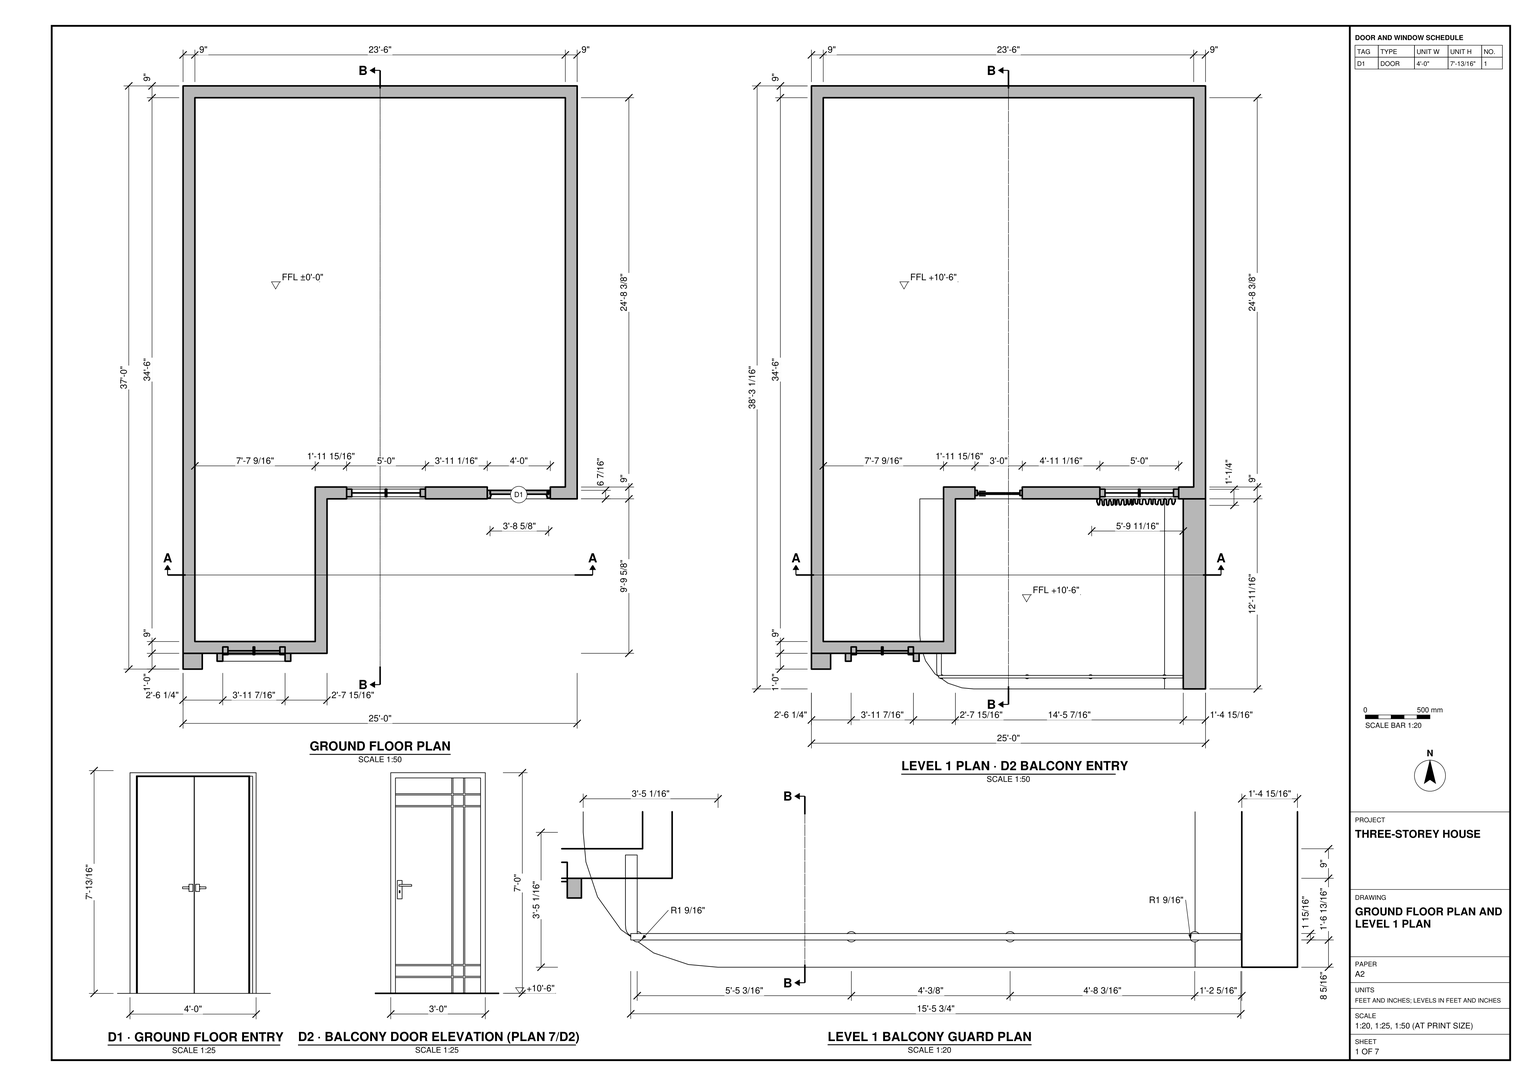
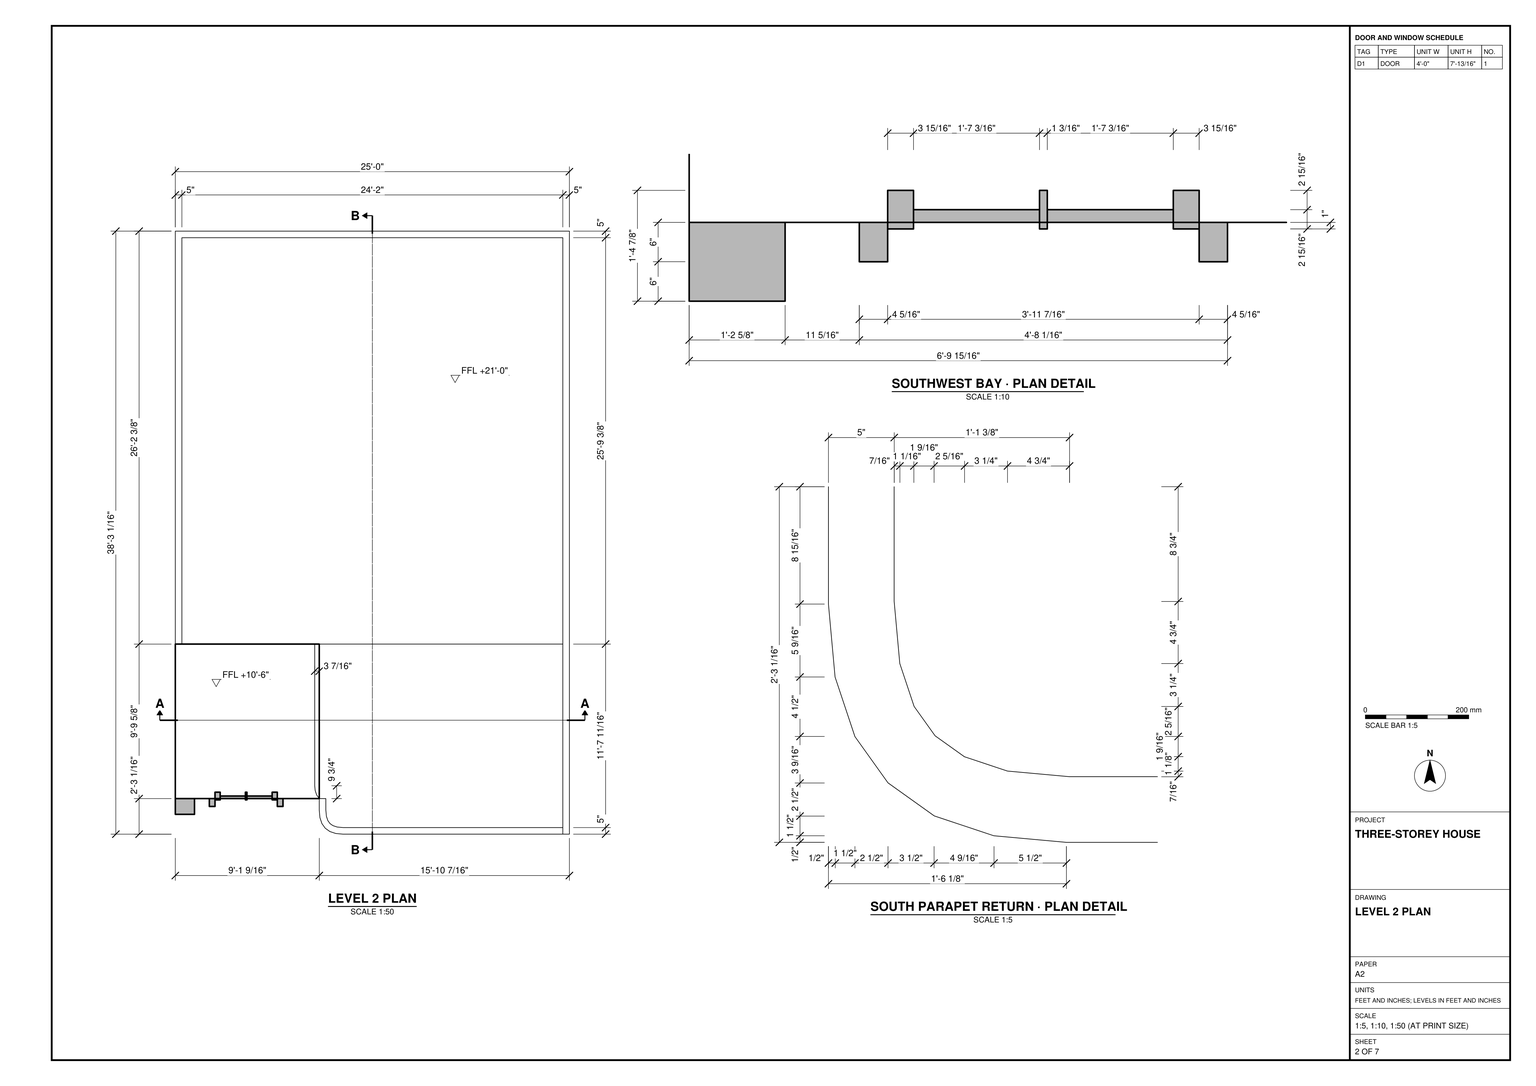
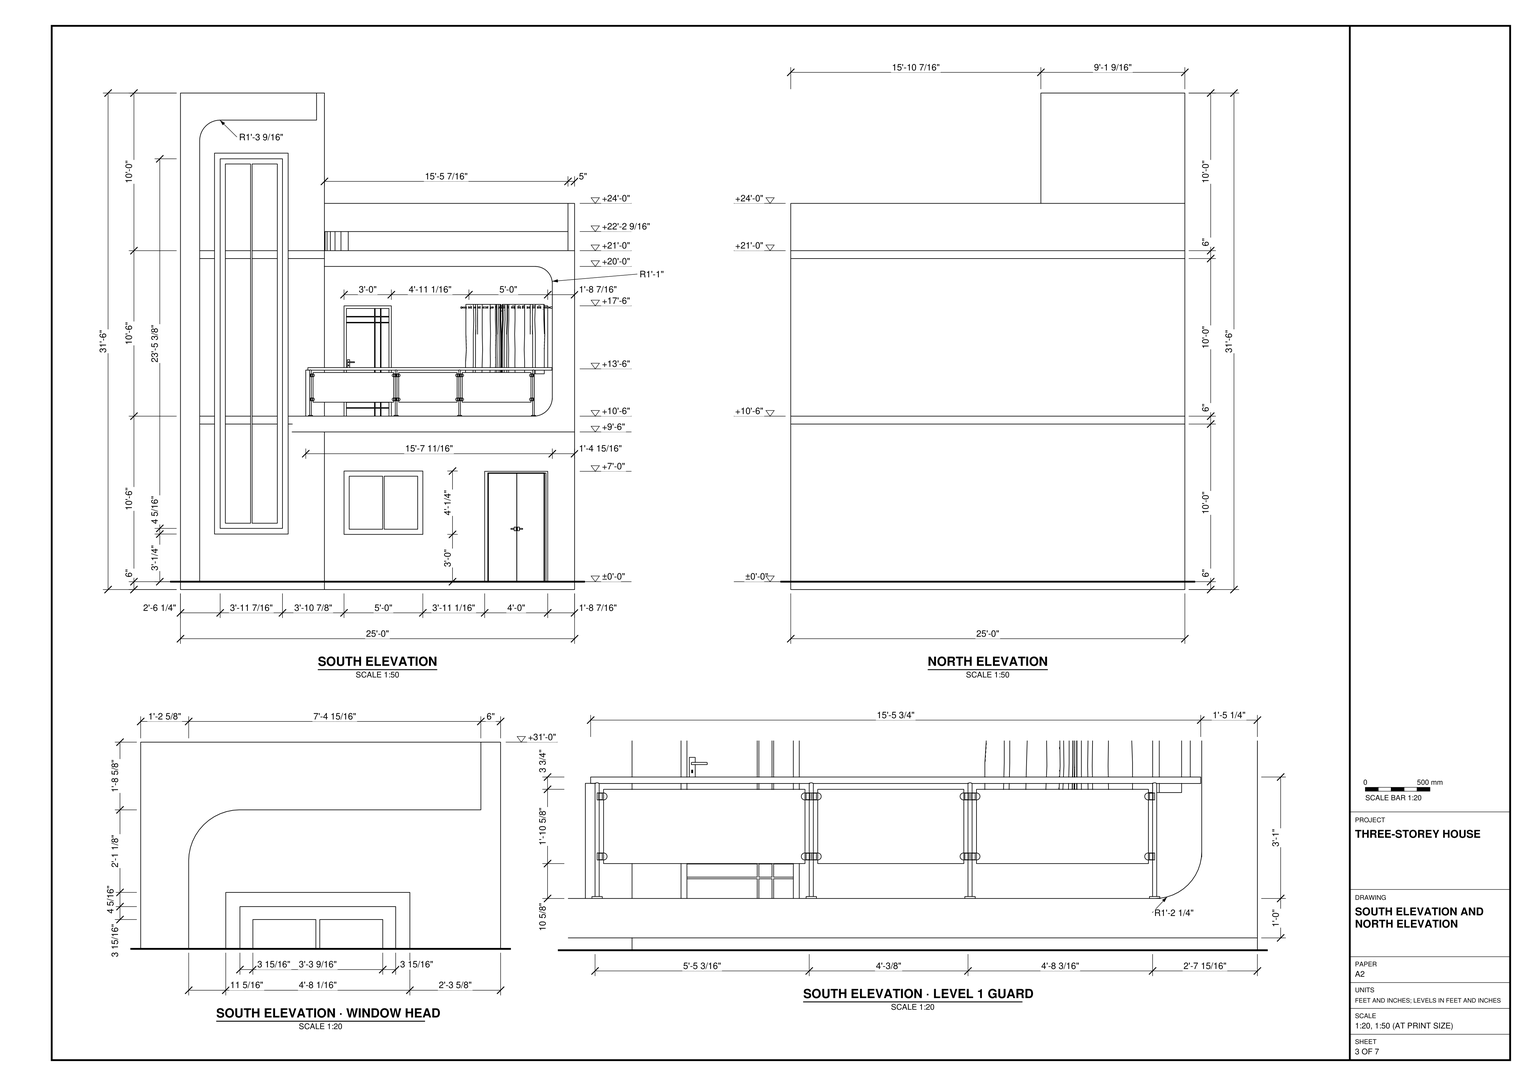
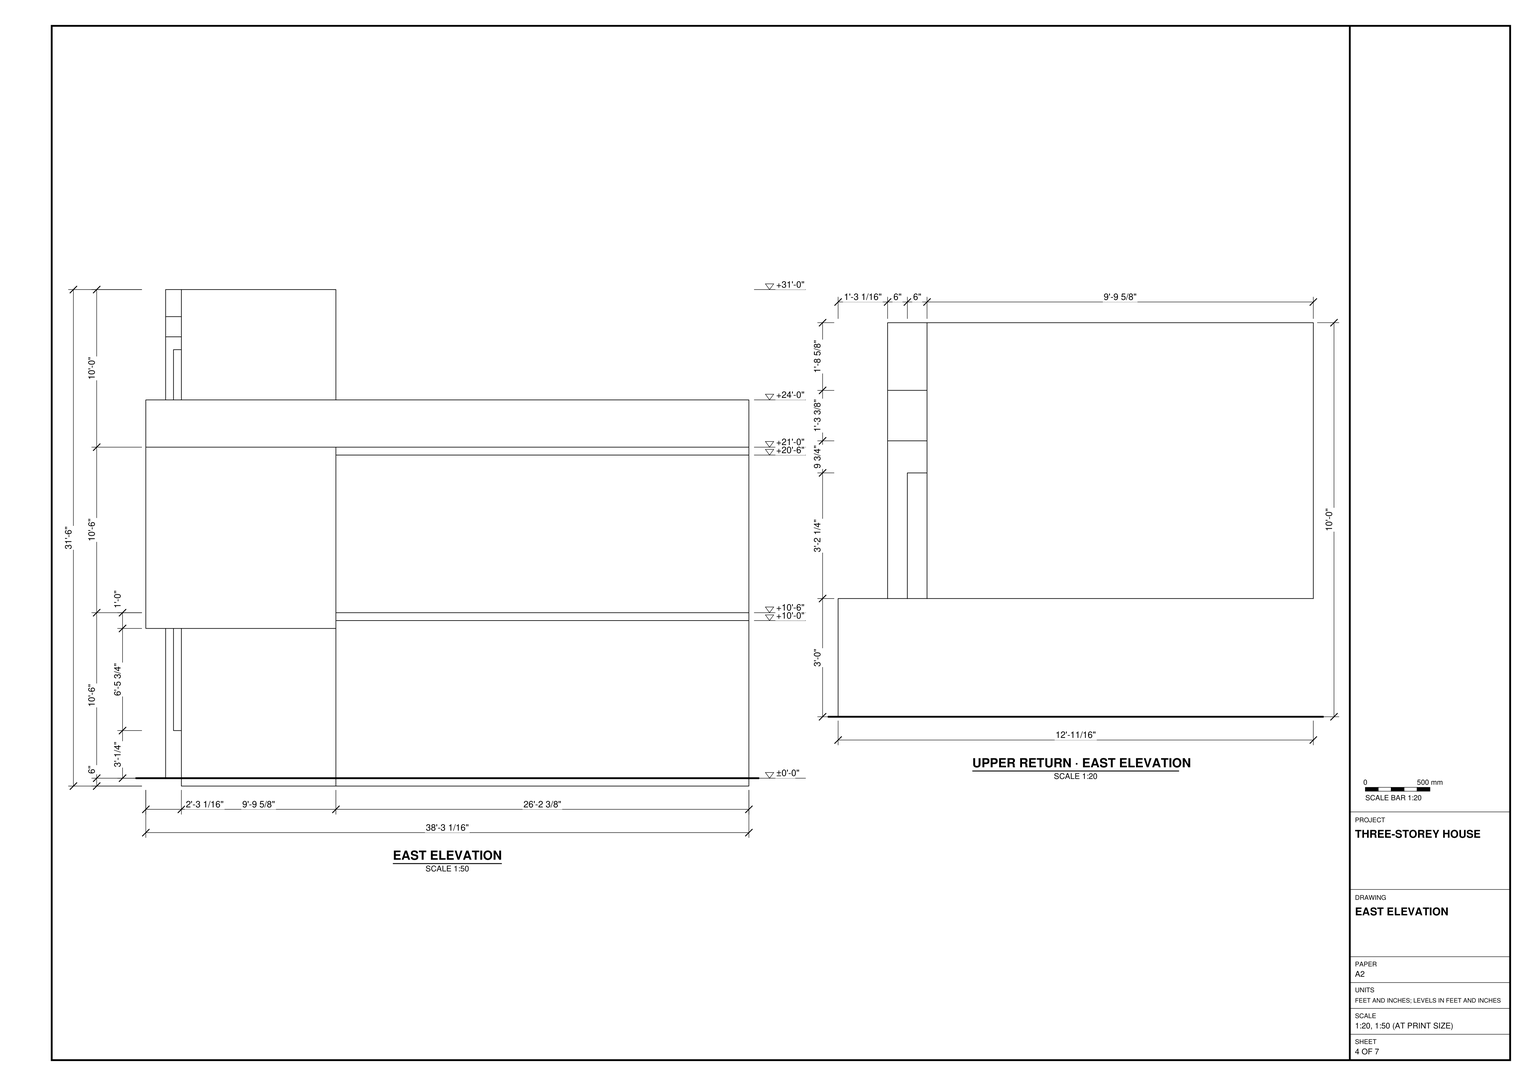
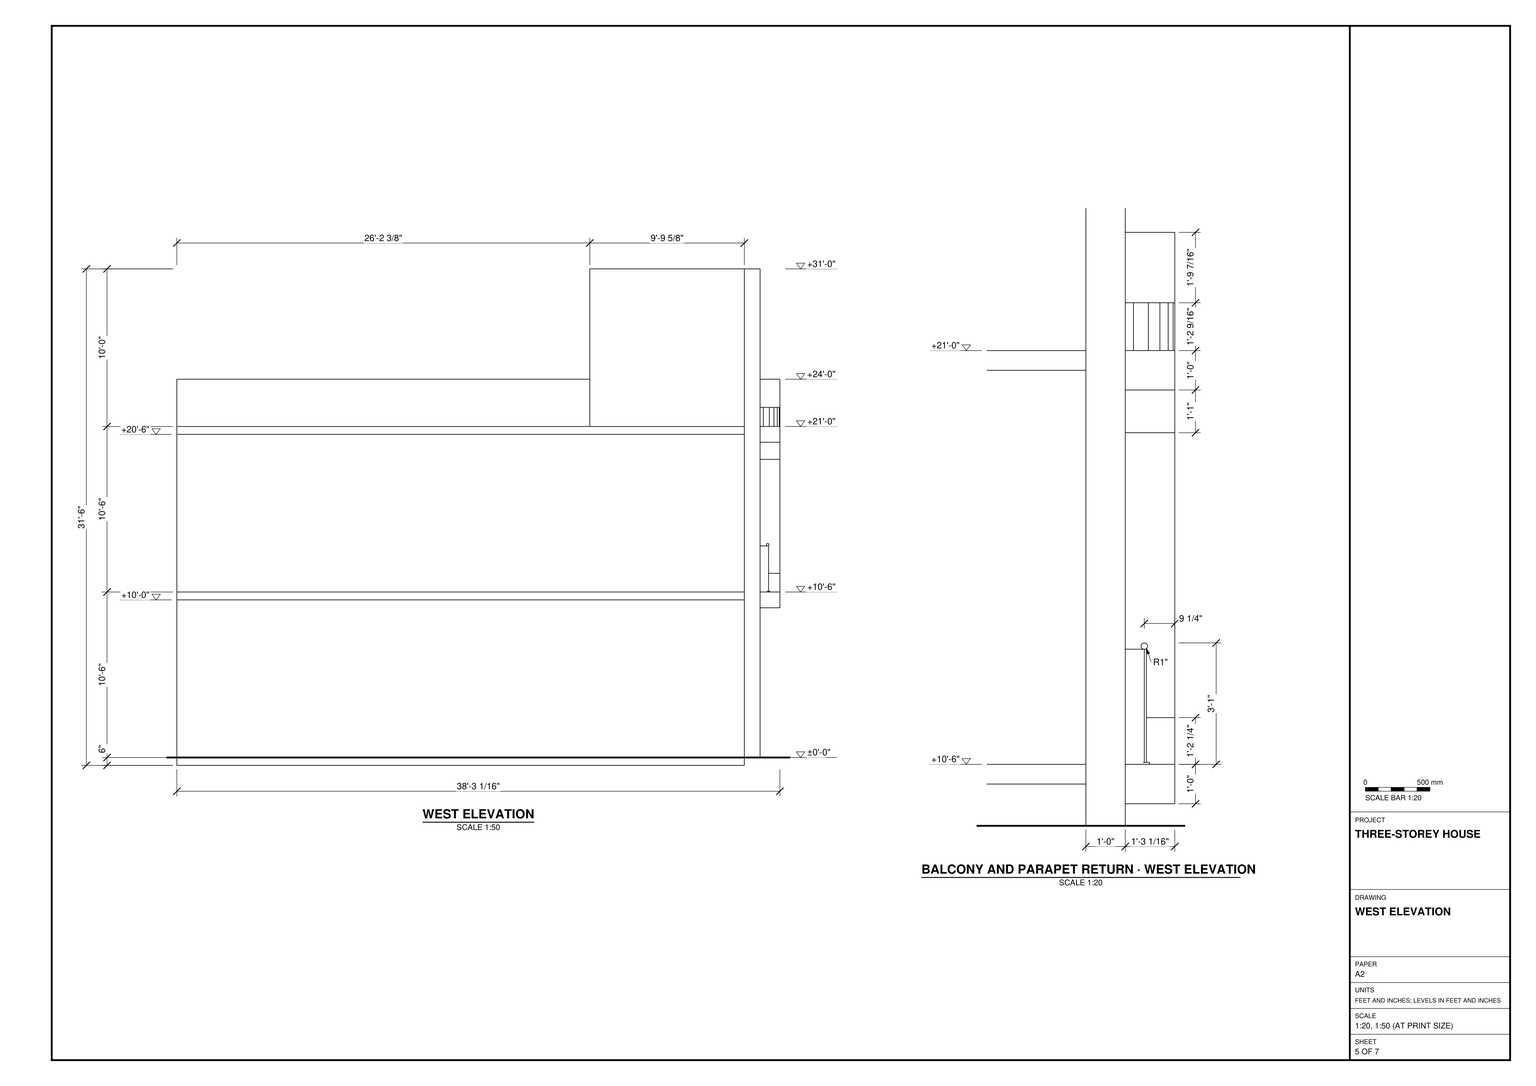
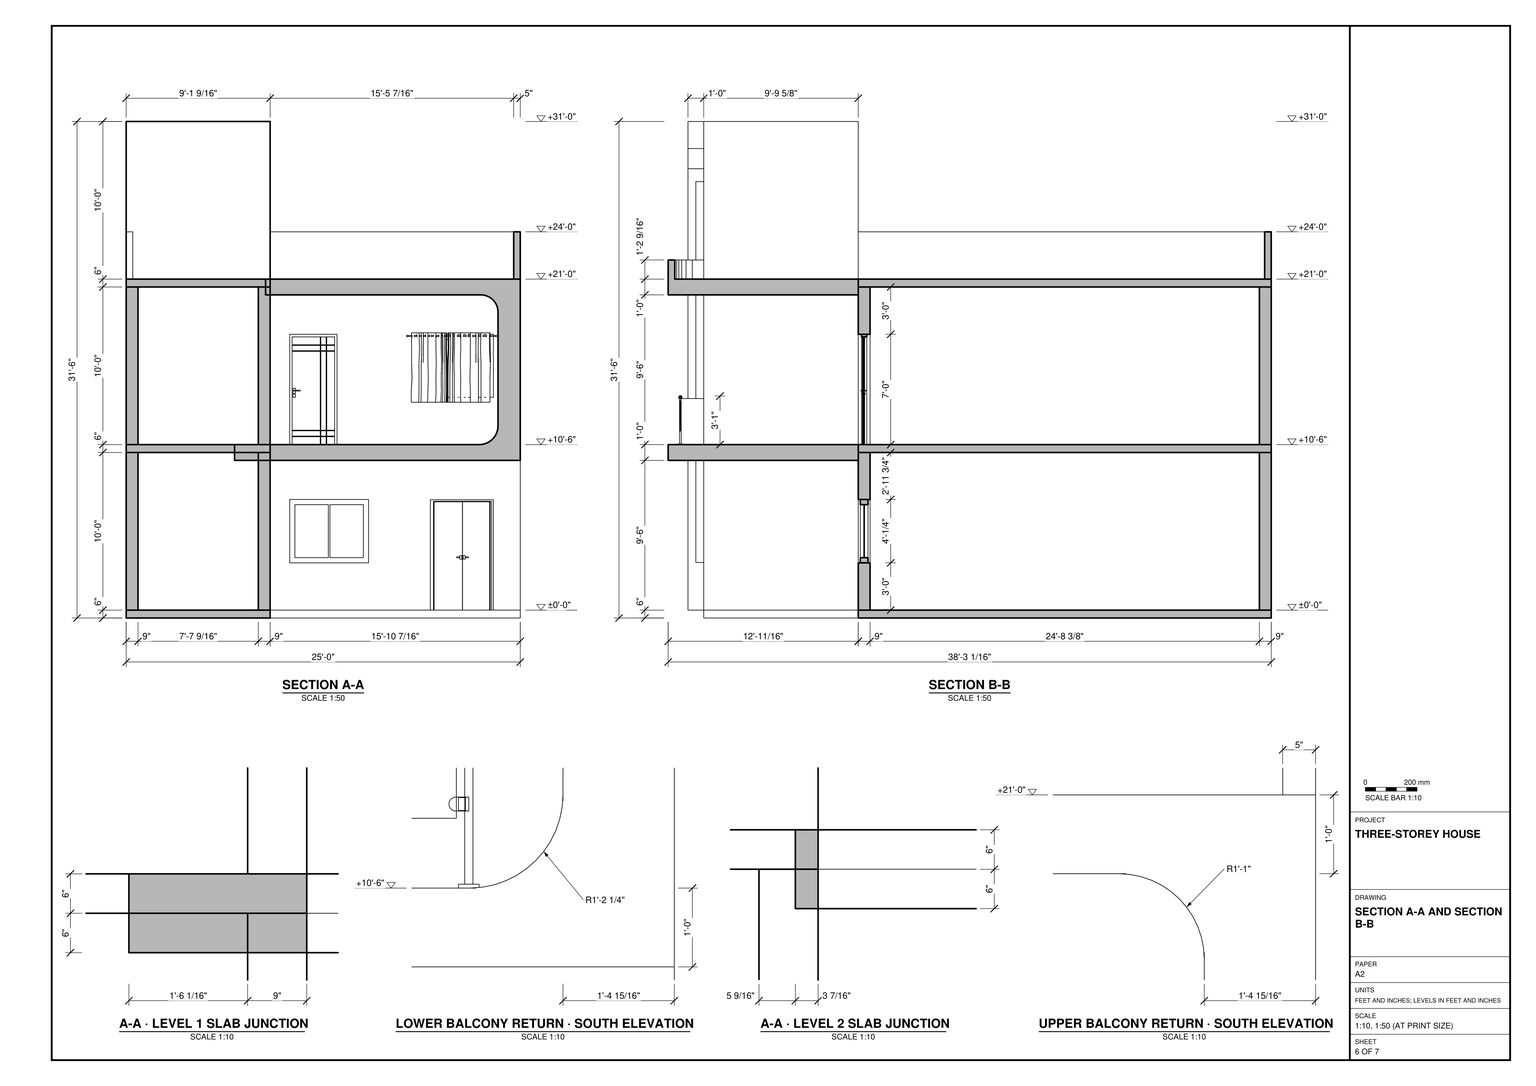
Build the three-storey house in SketchUp from task_files/diagram_01.pdf. Work in feet and inches. The overall model is 25'-0" wide by 38'-3 1/16" deep by 31'-6" high. Set the finished floor levels at ±0'-0", +10'-6" and +21'-0".

Use the plans to lay out the stepped ground-floor footprint. The narrow southwest bay projects beyond the recessed entrance wall. Model the walls at their drawn thicknesses, including the 9" main perimeter walls on the ground floor and level 1. Fit the double entry door and the adjacent window beneath the balcony. In the southwest bay, carry the tall divided window across the floor lines and reproduce the surround with its rounded inside corner at the head.

Model the floor slabs, the projecting level 1 balcony and its guard with posts, infill panels and a continuous top rail. Place the balcony door to the left of the curtained opening when viewed from the south. Follow the upper plan for the flat roof and curved south parapet return, keeping the southwest bay above the adjoining parapet. Decor and loose items shown may be represented by any suitable library components.

Keep shell elements such as walls, slabs and roof, and each furniture or joinery piece shown, in separate groups or components. Use components for repeated parts. Save one SketchUp model as output_files/three_storey_house_with_south_balcony_and_window_bay.skp.

# SketchUp Ruby script. Lengths in inches.
U = 1.inch
M = Sketchup.active_model
def pt(a) = Geom::Point3d.new(a.map { |v| v * U })
def face(e, loops, mat)
  f = e.add_face(loops[0].map { |a| pt(a) })
  loops[1..].each { |l| e.add_face(l.map { |a| pt(a) }).erase! }
  f.material = f.back_material = mat if mat
  f
end
# faces: each face lists its corners as indices into pts; further lists are holes
def faces(e, pts, list, mat = nil) = list.each { |f| face(e, (f[0].is_a?(Array) ? f : [f]).map { |l| l.map { |i| pts[i] } }, mat) }
# xy, xz, yz: faces in a plane at the given z, y or x. An outline is a flat list of corners, or four numbers for a rectangle; further outlines are holes
def ring(l) = l.size == 4 ? [[l[0], l[1]], [l[2], l[1]], [l[2], l[3]], [l[0], l[3]]] : l.each_slice(2).to_a
def flat(e, list, mat, &to3) = list.each { |f| face(e, (f[0].is_a?(Array) ? f : [f]).map { |l| ring(l).map { |u, v| to3.(u, v) } }, mat) }
def xy(e, z, list, mat = nil) = flat(e, list, mat) { |x, y| [x, y, z] }
def xz(e, y, list, mat = nil) = flat(e, list, mat) { |x, z| [x, y, z] }
def yz(e, x, list, mat = nil) = flat(e, list, mat) { |y, z| [x, y, z] }
def lines(e, pts, list) = list.each { |a, b| e.add_line(pt(pts[a]), pt(pts[b])) }
# prism: a flat outline (further loops are holes) pulled along v
def prism(e, loops, v, mat = nil)
  f = face(e, loops, mat); d = Geom::Vector3d.new(v.map { |x| x * U })
  f.pushpull(f.normal.samedirection?(d) ? d.length : -d.length)
end
def box(e, o, s, mat = nil) = prism(e, [[o, [o[0] + s[0], o[1], o[2]], [o[0] + s[0], o[1] + s[1], o[2]], [o[0], o[1] + s[1], o[2]]]], [0, 0, s[2]], mat)
def at(x, y, z, deg = 0) = Geom::Transformation.translation(pt([x, y, z])) * Geom::Transformation.rotation(ORIGIN, Z_AXIS, deg.degrees)
def axes(o, x, y, z) = Geom::Transformation.new([*x, 0, *y, 0, *z, 0, *pt(o).to_a, 1])
def part(name) = M.definitions.add(name)
# library, detail: a bought-in or finely detailed component or shape, given as its bounding box
def library(name, o, s) = part(name).tap { |d| box(d.entities, o, s) }
def detail(e, o, s) = box(e.add_group.entities, o, s)
def put(e, d, t, mat = nil) = e.add_instance(d, t).tap { |i| i.material = mat if mat }
def group(e, t, mat = nil) = e.add_group.tap { |g| g.transformation = t; g.material = mat if mat }.entities
root = M.entities
M.materials.add("[Color C05]").color = [255, 127, 0]
M.materials.add("[Color M03]").color = [170, 170, 170]
M.materials.add("[Color M09]").color = [0, 0, 0]
M.materials.add("[Color_B21]").color = [51, 12, 0]
M.materials.add("[Color_L25]").color = [117, 101, 92]
M.materials.add("[Granite Brown]").color = [126, 104, 91]
M.materials.add("[Granite Light Gray]").color = [149, 148, 144]
M.materials.add("[Mirror 01]").color = [185, 185, 185]
M.materials.add("[Translucent Glass Blue]").color = [100, 149, 237]
M.materials["[Translucent Glass Blue]"].alpha = 0.5
M.materials.add("[Wood Cherry Original]").color = [152, 86, 42]
c1 = library("Untitled",[0,0,0],[36,4.39,84])
c2 = library("CURTAIN\#1",[-0.6,-7.68,-83.58],[11.58,83.5,83.58])
c3 = part("Group17\#2")
xy(c3.entities,0,[[-26.0625,-20.0625,-0.59,20.0625],[0.59,-20.0625,26.0625,20.0625]])
c4 = part("Group16\#1")
prism(c4.entities,[[[-30,-24,0],[-30,24,0],[30,24,0],[30,-24,0]],[[-0.59,20.0625,0],[-26.0625,20.0625,0],[-26.0625,-20.0625,0],[-0.59,-20.0625,0]],[[0.59,-20.0625,0],[26.0625,-20.0625,0],[26.0625,20.0625,0],[0.59,20.0625,0]]],[0,0,5.875])
put(c4.entities,c3,at(0,0,2.9375),"[Translucent Glass Blue]")
c5 = part("Group17\#3")
xy(c5.entities,0,[[-26.0625,-20.18,-0.59,20.18],[0.59,-20.18,26.0625,20.18]])
c6 = part("Group16\#2")
prism(c6.entities,[[[-30,-24.12,0],[-30,24.12,0],[30,24.12,0],[30,-24.12,0]],[[0.59,20.18,0],[0.59,-20.18,0],[26.0625,-20.18,0],[26.0625,20.18,0]],[[-0.59,20.18,0],[-26.0625,20.18,0],[-26.0625,-20.18,0],[-0.59,-20.18,0]]],[0,0,5.875])
put(c6.entities,c5,at(0,0,2.9375),"[Translucent Glass Blue]")
c7 = part("Door frame")
xy(c7.entities,0,[[0,0,0,3.9375,1.97,3.9375,1.97,1.97,2.36,1.97,2.36,1.18,2.17,1.18,2.17,0.85,1.97,0.85,1.97,0],[37.73,0,37.73,0.85,37.53,0.85,37.53,1.18,37.34,1.18,37.34,1.97,37.73,1.97,37.73,3.9375,39.7,3.9375,39.7,0]])
xy(c7.entities,82.45,[[2.36,1.18,37.34,1.97]])
xy(c7.entities,82.64,[[2.17,0.85,37.53,1.18]])
xy(c7.entities,82.84,[[1.97,0,37.73,0.85],[1.97,1.97,37.73,3.9375]])
xy(c7.entities,84.81,[[0,0,39.7,3.9375]],"[Color_B21]")
xz(c7.entities,0,[[0,0,1.97,0,1.97,82.84,37.73,82.84,37.73,0,39.7,0,39.7,84.81,0,84.81]],"[Color_L25]")
xz(c7.entities,0.85,[[1.97,0,2.17,0,2.17,82.64,37.53,82.64,37.53,0,37.73,0,37.73,82.84,1.97,82.84]],"[Color_L25]")
xz(c7.entities,1.18,[[2.17,0,2.36,0,2.36,82.45,37.34,82.45,37.34,0,37.53,0,37.53,82.64,2.17,82.64]],"[Color_B21]")
xz(c7.entities,1.97,[[1.97,0,1.97,82.84,37.73,82.84,37.73,0,37.34,0,37.34,82.45,2.36,82.45,2.36,0]])
xz(c7.entities,3.9375,[[0,0,0,84.81,39.7,84.81,39.7,0,37.73,0,37.73,82.84,1.97,82.84,1.97,0]],"[Color_B21]")
yz(c7.entities,0,[[0,0,3.9375,84.81]],"[Color_B21]")
yz(c7.entities,1.97,[[1.97,0,3.9375,82.84]])
yz(c7.entities,1.97,[[0,0,0.85,82.84]],"[Color_L25]")
yz(c7.entities,2.17,[[0.85,0,1.18,82.64]],"[Color_L25]")
yz(c7.entities,2.36,[[1.18,0,1.97,82.45]],"[Color_B21]")
yz(c7.entities,37.34,[[1.18,0,1.97,82.45]],"[Color_B21]")
yz(c7.entities,37.53,[[0.85,0,1.18,82.64]],"[Color_L25]")
yz(c7.entities,37.73,[[1.97,0,3.9375,82.84]])
yz(c7.entities,37.73,[[0,0,0.85,82.84]],"[Color_L25]")
yz(c7.entities,39.7,[[0,0,3.9375,84.81]],"[Color_B21]")
p = [[2.13,0.01,0],[2.13,0.01,82.68],[37.57,0.01,82.68],[37.57,0.01,0]]
lines(c7.entities,p,[[0,1],[1,2],[2,3]])
c8 = part("Elegant door(double)")
p = [[77.86,31.43,0],[42.82,31.43,0],[38.88,31.43,0]]
lines(c8.entities,p,[[0,1],[1,2]])
put(c8.entities,c7,axes([38.88,29.47,0],[1.93222,0,0],[0,1,0],[0,0,1]),"[Color_B21]")
g1 = group(c8.entities,at(77.86,29.07,0))
xy(g1,0,[[0,2.36,35.76,4.33]])
xy(g1,38.8,[[1.3,0,1.36,2.36],[1.36,0,3.29,2.36]],"[Color_L25]")
xy(g1,39.63,[[3.29,0.09,3.54,0.79]],"[Color_L25]")
xy(g1,39.85,[[3.54,0.09,7.14,0.79]],"[Color_L25]")
xy(g1,39.86,[[7.15,0.09,7.16,0.79]],"[Color_L25]")
xy(g1,40.55,[[7.15,0.09,7.17,0.79]],"[Color_L25]")
xy(g1,40.5625,[[3.53,0.09,7.11,0.79],[7.11,0.09,7.125,0.79]],"[Color_L25]")
xy(g1,40.8125,[[3.29,0.09,3.53,0.79]],"[Color_L25]")
xy(g1,41.55,[[1.35,0,1.41,2.36],[1.41,0,3.29,2.36]],"[Color_L25]")
xy(g1,82.84,[[0,2.36,35.76,4.33]])
xz(g1,0,[[1.3,38.8,3.29,38.8,3.29,41.55,1.35,41.55,1.28,41.54,1.23,41.52,1.17,41.49,1.07,41.41,1.03,41.37,0.99,41.31,0.97,41.26,0.95,41.2,0.93,41.08,0.93,39.17,0.95,39.11,0.96,39.0625,0.99,39.01,1.02,38.96,1.06,38.92,1.1,38.89,1.14,38.85,1.19,38.83,1.25,38.8125]],"[Color_L25]")
xz(g1,0.09,[[3.29,39.63,3.54,39.63,3.54,39.85,7.14,39.85,7.15,39.86,7.16,39.86,7.18,39.87,7.1875,39.875,7.2,39.88,7.21,39.89,7.22,39.91,7.22,39.92,7.23,39.93,7.23,40.47,7.22,40.49,7.2,40.51,7.19,40.53,7.17,40.55,7.15,40.55,7.14,40.56,7.125,40.5625,3.53,40.5625,3.53,40.8125,3.29,40.8125]],"[Color_L25]")
xz(g1,0.79,[[3.29,39.63,3.29,40.8125,3.53,40.8125,3.53,40.5625,7.125,40.5625,7.14,40.56,7.15,40.55,7.17,40.55,7.19,40.53,7.2,40.51,7.22,40.49,7.23,40.47,7.23,39.93,7.22,39.92,7.22,39.91,7.21,39.89,7.2,39.88,7.1875,39.875,7.18,39.87,7.16,39.86,7.15,39.86,7.14,39.85,3.54,39.85,3.54,39.63]],"[Color_L25]")
xz(g1,2.36,[[[0,0,35.76,82.84],[0.93,38.8,3.29,41.55]],[0.93,38.8,1.36,38.8,1.3,38.8,1.25,38.8125,1.19,38.83,1.14,38.85,1.1,38.89,1.06,38.92,1.02,38.96,0.99,39.01,0.96,39.0625,0.95,39.11,0.93,39.17,0.93,39.22],[0.93,41.08,0.95,41.2,0.97,41.26,0.99,41.31,1.03,41.37,1.07,41.41,1.17,41.49,1.23,41.52,1.28,41.54,1.35,41.55,1.41,41.55,0.93,41.55]],"[Color_L25]")
xz(g1,4.33,[[0,0,35.76,82.84]])
yz(g1,0,[[2.36,0,4.33,82.84]])
yz(g1,0.93,[[0,39.17,2.36,39.22],[0,39.22,2.36,41.08]],"[Color_L25]")
yz(g1,3.29,[[[0,38.8,2.36,41.55],[0.09,39.63,0.79,40.8125]]],"[Color_L25]")
yz(g1,3.53,[[0.09,40.5625,0.79,40.8125]],"[Color_L25]")
yz(g1,3.54,[[0.09,39.63,0.79,39.85]],"[Color_L25]")
yz(g1,7.22,[[0.09,39.91,0.79,39.92]],"[Color_L25]")
yz(g1,7.23,[[0.09,39.93,0.79,39.94],[0.09,39.94,0.79,40.4375],[0.09,40.4375,0.79,40.46],[0.09,40.46,0.79,40.47]],"[Color_L25]")
yz(g1,35.76,[[2.36,0,4.33,82.84]])
p = [[1.19,0,38.83],[1.14,0,38.85],[1.14,2.36,38.85],[1.19,2.36,38.83],[1.3,0,38.8],[1.25,0,38.8125],
  [1.25,2.36,38.8125],[1.3,2.36,38.8],[1.06,0,38.92],[1.02,0,38.96],[1.02,2.36,38.96],[1.06,2.36,38.92],
  [1.1,0,38.89],[1.1,2.36,38.89],[0.99,0,39.01],[0.99,2.36,39.01],[0.96,0,39.0625],[0.96,2.36,39.0625],
  [0.95,0,39.11],[0.95,2.36,39.11],[0.93,0,39.17],[0.93,2.36,39.17],[7.15,0.09,39.86],[7.14,0.09,39.85],
  [7.14,0.79,39.85],[7.15,0.79,39.86],[7.22,0.09,39.91],[7.21,0.09,39.89],[7.21,0.79,39.89],[7.22,0.79,39.91],
  [7.2,0.09,39.88],[7.2,0.79,39.88],[7.1875,0.09,39.875],[7.1875,0.79,39.875],[7.18,0.09,39.87],[7.18,0.79,39.87],
  [7.16,0.09,39.86],[7.16,0.79,39.86],[7.23,0.09,39.93],[7.22,0.09,39.92],[7.22,0.79,39.92],[7.23,0.79,39.93],
  [7.17,0.09,40.55],[7.18,0.09,40.54],[7.18,0.79,40.54],[7.17,0.79,40.55],[7.19,0.09,40.53],[7.19,0.79,40.53],
  [7.2,0.09,40.51],[7.2,0.79,40.51],[7.21,0.09,40.5],[7.21,0.79,40.5],[7.22,0.09,40.49],[7.22,0.79,40.49],
  [7.23,0.09,40.47],[7.23,0.79,40.47],[7.125,0.09,40.5625],[7.14,0.09,40.56],[7.14,0.79,40.56],[7.125,0.79,40.5625],
  [7.15,0.09,40.55],[7.15,0.79,40.55],[0.93,0,41.08],[0.94,0,41.14],[0.94,2.36,41.14],[0.93,2.36,41.08],
  [0.95,0,41.2],[0.95,2.36,41.2],[0.97,0,41.26],[0.97,2.36,41.26],[0.99,0,41.31],[0.99,2.36,41.31],
  [1.03,0,41.37],[1.03,2.36,41.37],[1.07,0,41.41],[1.07,2.36,41.41],[1.12,0,41.45],[1.12,2.36,41.45],
  [1.17,0,41.49],[1.17,2.36,41.49],[1.23,0,41.52],[1.23,2.36,41.52],[1.28,0,41.54],[1.28,2.36,41.54],
  [1.35,0,41.55],[1.35,2.36,41.55],[0.16,0.41,82.68],[35.6,0.41,82.68],[35.6,0.41,0]]
faces(g1,p,[[0,1,2,3],[4,5,6,7],[5,0,3,6],[8,9,10,11],[1,12,13,2],[12,8,11,13],[9,14,15,10],[14,16,17,15],
  [16,18,19,17],[18,20,21,19],[22,23,24,25],[26,27,28,29],[27,30,31,28],[30,32,33,31],[32,34,35,33],[34,36,37,35],
  [38,39,40,41],[42,43,44,45],[43,46,47,44],[46,48,49,47],[48,50,51,49],[50,52,53,51],[52,54,55,53],[56,57,58,59],
  [57,60,61,58],[62,63,64,65],[63,66,67,64],[66,68,69,67],[68,70,71,69],[70,72,73,71],[72,74,75,73],[74,76,77,75],
  [76,78,79,77],[78,80,81,79],[80,82,83,81],[82,84,85,83]],"[Color_L25]")
lines(g1,p,[[86,87],[87,88]])
g2 = group(c8.entities,at(78.05,29.07,0))
xy(g2,0,[[-35.76,2.36,0,4.33]])
xy(g2,38.8,[[-3.29,0,-1.36,2.36],[-1.36,0,-1.3,2.36]],"[Color_L25]")
xy(g2,39.63,[[-3.54,0.09,-3.29,0.79]],"[Color_L25]")
xy(g2,39.85,[[-7.14,0.09,-3.54,0.79]],"[Color_L25]")
xy(g2,39.86,[[-7.16,0.09,-7.15,0.79]],"[Color_L25]")
xy(g2,40.55,[[-7.17,0.09,-7.15,0.79]],"[Color_L25]")
xy(g2,40.5625,[[-7.125,0.09,-7.11,0.79],[-7.11,0.09,-3.53,0.79]],"[Color_L25]")
xy(g2,40.8125,[[-3.53,0.09,-3.29,0.79]],"[Color_L25]")
xy(g2,41.55,[[-3.29,0,-1.41,2.36],[-1.41,0,-1.35,2.36]],"[Color_L25]")
xy(g2,82.84,[[-35.76,2.36,0,4.33]])
xz(g2,0,[[-3.29,38.8,-3.29,41.55,-1.35,41.55,-1.28,41.54,-1.23,41.52,-1.17,41.49,-1.07,41.41,-1.03,41.37,-0.99,41.31,-0.97,41.26,-0.95,41.2,-0.93,41.08,-0.93,39.17,-0.95,39.11,-0.96,39.0625,-0.99,39.01,-1.02,38.96,-1.06,38.92,-1.1,38.89,-1.14,38.85,-1.19,38.83,-1.25,38.8125,-1.3,38.8]],"[Color_L25]")
xz(g2,0.09,[[-3.54,39.63,-3.54,39.85,-7.14,39.85,-7.15,39.86,-7.16,39.86,-7.18,39.87,-7.1875,39.875,-7.2,39.88,-7.21,39.89,-7.22,39.91,-7.22,39.92,-7.23,39.93,-7.23,40.47,-7.22,40.49,-7.2,40.51,-7.19,40.53,-7.17,40.55,-7.15,40.55,-7.14,40.56,-7.125,40.5625,-3.53,40.5625,-3.53,40.8125,-3.29,40.8125,-3.29,39.63]],"[Color_L25]")
xz(g2,0.79,[[-3.54,39.63,-3.29,39.63,-3.29,40.8125,-3.53,40.8125,-3.53,40.5625,-7.125,40.5625,-7.14,40.56,-7.15,40.55,-7.17,40.55,-7.19,40.53,-7.2,40.51,-7.22,40.49,-7.23,40.47,-7.23,39.93,-7.22,39.92,-7.22,39.91,-7.21,39.89,-7.2,39.88,-7.1875,39.875,-7.18,39.87,-7.16,39.86,-7.15,39.86,-7.14,39.85,-3.54,39.85]],"[Color_L25]")
xz(g2,2.36,[[[-35.76,0,0,82.84],[-3.29,38.8,-0.93,41.55]],[-1.36,38.8,-1.3,38.8,-1.25,38.8125,-1.19,38.83,-1.14,38.85,-1.1,38.89,-1.06,38.92,-1.02,38.96,-0.99,39.01,-0.96,39.0625,-0.95,39.11,-0.93,39.17,-0.93,39.22,-0.93,38.8],[-0.93,41.08,-0.95,41.2,-0.97,41.26,-0.99,41.31,-1.03,41.37,-1.07,41.41,-1.17,41.49,-1.23,41.52,-1.28,41.54,-1.35,41.55,-1.41,41.55,-0.93,41.55]],"[Color_L25]")
xz(g2,4.33,[[-35.76,0,0,82.84]])
yz(g2,-35.76,[[2.36,0,4.33,82.84]])
yz(g2,-7.23,[[0.09,39.93,0.79,39.94],[0.09,39.94,0.79,40.4375],[0.09,40.4375,0.79,40.46],[0.09,40.46,0.79,40.47]],"[Color_L25]")
yz(g2,-7.22,[[0.09,39.91,0.79,39.92]],"[Color_L25]")
yz(g2,-3.54,[[0.09,39.63,0.79,39.85]],"[Color_L25]")
yz(g2,-3.53,[[0.09,40.5625,0.79,40.8125]],"[Color_L25]")
yz(g2,-3.29,[[[0,38.8,2.36,41.55],[0.09,39.63,0.79,40.8125]]],"[Color_L25]")
yz(g2,-0.93,[[0,39.17,2.36,39.22],[0,39.22,2.36,41.08]],"[Color_L25]")
yz(g2,0,[[2.36,0,4.33,82.84]])
p = [[-1.3,0,38.8],[-1.25,0,38.8125],[-1.25,2.36,38.8125],[-1.3,2.36,38.8],[-1.19,0,38.83],[-1.19,2.36,38.83],
  [-1.14,0,38.85],[-1.14,2.36,38.85],[-1.1,0,38.89],[-1.1,2.36,38.89],[-1.06,0,38.92],[-1.06,2.36,38.92],
  [-1.02,0,38.96],[-1.02,2.36,38.96],[-0.99,0,39.01],[-0.99,2.36,39.01],[-0.96,0,39.0625],[-0.96,2.36,39.0625],
  [-0.95,0,39.11],[-0.95,2.36,39.11],[-0.93,0,39.17],[-0.93,2.36,39.17],[-7.22,0.09,39.91],[-7.21,0.09,39.89],
  [-7.21,0.79,39.89],[-7.22,0.79,39.91],[-7.2,0.09,39.88],[-7.2,0.79,39.88],[-7.1875,0.09,39.875],[-7.1875,0.79,39.875],
  [-7.18,0.09,39.87],[-7.18,0.79,39.87],[-7.16,0.09,39.86],[-7.16,0.79,39.86],[-7.15,0.09,39.86],[-7.14,0.09,39.85],
  [-7.14,0.79,39.85],[-7.15,0.79,39.86],[-7.23,0.09,39.93],[-7.22,0.09,39.92],[-7.22,0.79,39.92],[-7.23,0.79,39.93],
  [-7.17,0.09,40.55],[-7.18,0.09,40.54],[-7.18,0.79,40.54],[-7.17,0.79,40.55],[-7.19,0.09,40.53],[-7.19,0.79,40.53],
  [-7.2,0.09,40.51],[-7.2,0.79,40.51],[-7.21,0.09,40.5],[-7.21,0.79,40.5],[-7.22,0.09,40.49],[-7.22,0.79,40.49],
  [-7.23,0.09,40.47],[-7.23,0.79,40.47],[-7.14,0.09,40.56],[-7.15,0.09,40.55],[-7.15,0.79,40.55],[-7.14,0.79,40.56],
  [-7.125,0.09,40.5625],[-7.125,0.79,40.5625],[-0.93,0,41.08],[-0.94,0,41.14],[-0.94,2.36,41.14],[-0.93,2.36,41.08],
  [-0.95,0,41.2],[-0.95,2.36,41.2],[-0.97,0,41.26],[-0.97,2.36,41.26],[-0.99,0,41.31],[-0.99,2.36,41.31],
  [-1.03,0,41.37],[-1.03,2.36,41.37],[-1.07,0,41.41],[-1.07,2.36,41.41],[-1.12,0,41.45],[-1.12,2.36,41.45],
  [-1.23,0,41.52],[-1.28,0,41.54],[-1.28,2.36,41.54],[-1.23,2.36,41.52],[-1.35,0,41.55],[-1.35,2.36,41.55],
  [-1.17,0,41.49],[-1.17,2.36,41.49]]
faces(g2,p,[[0,1,2,3],[1,4,5,2],[4,6,7,5],[6,8,9,7],[8,10,11,9],[10,12,13,11],[12,14,15,13],[14,16,17,15],
  [16,18,19,17],[18,20,21,19],[22,23,24,25],[23,26,27,24],[26,28,29,27],[28,30,31,29],[30,32,33,31],[34,35,36,37],
  [38,39,40,41],[42,43,44,45],[43,46,47,44],[46,48,49,47],[48,50,51,49],[50,52,53,51],[52,54,55,53],[56,57,58,59],
  [60,56,59,61],[62,63,64,65],[63,66,67,64],[66,68,69,67],[68,70,71,69],[70,72,73,71],[72,74,75,73],[74,76,77,75],
  [78,79,80,81],[79,82,83,80],[76,84,85,77],[84,78,81,85]],"[Color_L25]")
c9 = library("Group\#11",[0,0,0],[185.89,3.15,36.98])
c10 = part("Group62\#2")
xy(c10.entities,0,[[-19.77,-136.74,-0.59,136.74],[0.59,-136.74,19.77,136.74]])
c11 = part("Group61\#1")
prism(c11.entities,[[[23.71,-140.68,0],[-23.71,-140.68,0],[-23.71,140.68,0],[23.71,140.68,0]],[[-19.77,136.74,0],[-19.77,-136.74,0],[-0.59,-136.74,0],[-0.59,136.74,0]],[[0.59,-136.74,0],[19.77,-136.74,0],[19.77,136.74,0],[0.59,136.74,0]]],[0,0,5.875],"[Color M09]")
put(c11.entities,c10,at(0,0,2.9375))
c12 = part("Group64\#1")
prism(c12.entities,[[[2251.3125,3792.55,252],[1961.3125,3792.55,252],[1961.3125,3483.18,252],[1956.3125,3483.18,252],[1956.3125,3797.55,252],[2256.3125,3797.55,252],[2256.3125,3338.47,252],[2251.3125,3338.47,252]]],[0,0,36])
xy(root,0,[[0,15.08,14.61,27.08]],"[Granite Light Gray]")
xy(root,36.26,[[25.9,21.08,81.96,27.08]],"[Granite Brown]")
xy(root,40.58,[[30.22,21.08,77.65,26.08]],"[Granite Brown]")
xy(root,114,[[123.57,0,114.57,0.82,103.92,4.37,93.98,11.47,86.87,21.41,83.32,32.0625,82.51,41.0625,82.51,144.7,300,144.7,300,0]])
xy(root,126,[[123.57,0,268.83,0,268.83,144.7,82.51,144.7,82.51,41.0625,83.32,32.0625,86.87,21.41,93.98,11.47,103.92,4.37,114.57,0.82]])
xy(root,240,[[127.71,0,122.17,0.5,117.64,2.01,114.12,4.53,111.6,8.06,110.09,12.59,109.59,18.125,109.59,27.08,107.57,29.9,106.45,33.26,106.12,36.85,106.12,144.7,270.03,144.7,270.03,0]])
xy(root,252,[[295,0,300,0,300,144.7,106.12,144.7,106.12,36.85,106.45,33.26,107.57,29.9,109.59,27.08,114.59,27.08,114.59,18.35,115.02,13.62,116.1,10.35,117.7,8.12,119.94,6.52,123.2,5.43,127.9375,5,295,5]])
xy(root,266.5625,[[127.71,0,295,0,295,5,127.9375,5,123.2,5.43,119.94,6.52,117.7,8.12,116.1,10.35,115.02,13.62,114.59,18.35,114.59,27.08,109.59,27.08,109.59,18.125,110.09,12.59,111.6,8.06,114.12,4.53,117.64,2.01,122.17,0.5]],"[Color C05]")
xy(root,321.93,[[30.22,21.08,77.65,26.08]],"[Granite Brown]")
xy(root,326.25,[[25.9,21.08,81.96,27.08]],"[Granite Brown]")
xy(root,351.39,[[29.98,15.08,103.59,27.08]],"[Granite Light Gray]")
xy(root,372,[[0,15.08,103.59,27.08]],"[Granite Light Gray]")
xz(root,0,[[127.71,252,295,266.5625]],"[Color C05]")
xz(root,0,[[123.57,114,300,114,300,252,127.71,252,127.71,240,270.03,240,271.73,239.89,273.4,239.56,275.01,239.01,276.54,238.26,277.96,237.31,279.24,236.1875,280.36,234.91,281.31,233.49,282.06,231.96,282.61,230.35,282.9375,228.68,283.05,226.98,283.05,140.22,282.93,138.37,282.57,136.54,281.97,134.78,281.14,133.11,280.11,131.56,278.88,130.17,277.49,128.9375,275.9375,127.91,274.27,127.08,272.51,126.48,270.68,126.12,268.83,126,123.57,126]],"[Color M03]")
xz(root,5,[[127.9375,252,295,266.5625]],"[Color C05]")
xz(root,15.08,[[0,0,14.61,0,14.61,336.02,14.73,337.84,15.125,339.84,15.78,341.77,16.68,343.6,17.82,345.3,19.16,346.84,20.7,348.18,22.4,349.32,24.23,350.22,26.16,350.875,28.16,351.27,29.98,351.39,103.59,351.39,103.59,372,0,372]],"[Granite Light Gray]")
xz(root,21.08,[[[25.9,36.26,81.96,326.25],[30.22,40.58,77.65,321.93]]],"[Granite Brown]")
xz(root,27.08,[[0,0,0,372,103.59,372,103.59,351.39,29.98,351.39,28.16,351.27,26.16,350.875,24.23,350.22,22.4,349.32,20.7,348.18,19.16,346.84,17.82,345.3,16.68,343.6,15.78,341.77,15.125,339.84,14.73,337.84,14.61,336.02,14.61,0]])
xz(root,27.08,[[109.59,252,114.59,266.5625]],"[Color C05]")
xz(root,27.08,[[25.9,36.26,81.96,326.25]],"[Translucent Glass Blue]")
xz(root,144.7,[[82.51,114,283.05,124.45],[283.05,114,300,124.45],[82.51,124.45,283.05,126],[283.05,124.45,300,240],[268.83,126,270.68,126.12,272.51,126.48,274.27,127.08,275.9375,127.91,277.49,128.9375,278.88,130.17,280.11,131.56,281.14,133.11,281.97,134.78,282.57,136.54,282.93,138.37,283.05,140.22,283.05,126],
  [283.05,226.98,282.9375,228.68,282.61,230.35,282.06,231.96,281.31,233.49,280.36,234.91,279.24,236.1875,277.96,237.31,276.54,238.26,275.01,239.01,273.4,239.56,271.73,239.89,270.03,240,283.05,240],[106.12,240,145.65,252],[145.65,240,300,252]])
yz(root,0,[[15.08,0,27.08,372]],"[Granite Light Gray]")
yz(root,14.61,[[15.08,0,27.08,336.02]],"[Granite Light Gray]")
yz(root,25.9,[[21.08,36.26,27.08,326.25]],"[Granite Brown]")
yz(root,30.22,[[21.08,40.58,26.08,321.93]],"[Granite Brown]")
yz(root,77.65,[[21.08,40.58,26.08,321.93]],"[Granite Brown]")
yz(root,81.96,[[21.08,36.26,27.08,326.25]],"[Granite Brown]")
yz(root,82.51,[[41.0625,114,144.7,126]],"[Color M03]")
yz(root,98.95,[[9.28,126,27.08,161.0625]])
yz(root,103.59,[[15.08,351.39,27.08,372]],"[Granite Light Gray]")
yz(root,106.12,[[36.85,240,144.7,252]])
yz(root,109.59,[[18.125,252,27.08,266.5625]],"[Color C05]")
yz(root,109.59,[[18.125,240,27.08,252]],"[Color M03]")
yz(root,114.59,[[18.35,252,27.08,266.5625]],"[Color C05]")
yz(root,283.05,[[0,140.22,144.7,226.98]])
yz(root,295,[[0,252,5,266.5625]])
yz(root,300,[[0,114,144.7,252]])
p = [[123.57,0,114],[123.57,0,126],[114.57,0.82,126],[114.57,0.82,114],[103.92,4.37,126],[103.92,4.37,114],
  [93.98,11.47,114],[93.98,11.47,126],[86.87,21.41,126],[86.87,21.41,114],[83.32,32.0625,126],[83.32,32.0625,114],
  [82.51,41.0625,126],[82.51,41.0625,114],[268.83,0,126],[270.68,0,126.12],[270.68,144.7,126.12],[268.83,144.7,126],
  [272.51,0,126.48],[272.51,144.7,126.48],[274.27,0,127.08],[274.27,144.7,127.08],[275.9375,0,127.91],[275.9375,144.7,127.91],
  [277.49,0,128.9375],[277.49,144.7,128.9375],[278.88,0,130.17],[278.88,144.7,130.17],[280.11,0,131.56],[280.11,144.7,131.56],
  [281.14,0,133.11],[281.14,144.7,133.11],[281.97,0,134.78],[281.97,144.7,134.78],[282.57,0,136.54],[282.57,144.7,136.54],
  [282.93,0,138.37],[282.93,144.7,138.37],[283.05,0,140.22],[283.05,144.7,140.22],[283.05,0,226.98],[282.9375,0,228.68],
  [282.9375,144.7,228.68],[283.05,144.7,226.98],[282.61,0,230.35],[282.61,144.7,230.35],[282.06,0,231.96],[282.06,144.7,231.96],
  [281.31,0,233.49],[281.31,144.7,233.49],[280.36,0,234.91],[280.36,144.7,234.91],[279.24,0,236.1875],[279.24,144.7,236.1875],
  [277.96,0,237.31],[277.96,144.7,237.31],[276.54,0,238.26],[276.54,144.7,238.26],[275.01,0,239.01],[275.01,144.7,239.01],
  [273.4,0,239.56],[273.4,144.7,239.56],[271.73,0,239.89],[271.73,144.7,239.89],[270.03,0,240],[270.03,144.7,240],
  [122.17,0.5,252],[122.17,0.5,240],[127.71,0,240],[127.71,0,252],[117.64,2.01,252],[117.64,2.01,240],
  [114.12,4.53,252],[114.12,4.53,240],[111.6,8.06,252],[111.6,8.06,240],[110.09,12.59,252],[110.09,12.59,240],
  [109.59,18.125,252],[109.59,18.125,240],[109.59,27.08,252],[107.57,29.9,252],[107.57,29.9,240],[109.59,27.08,240],
  [106.45,33.26,252],[106.45,33.26,240],[106.12,36.85,252],[106.12,36.85,240],[127.71,0,266.5625],[122.17,0.5,266.5625],
  [117.64,2.01,266.5625],[114.12,4.53,266.5625],[111.6,8.06,266.5625],[127.9375,5,266.5625],[127.9375,5,252],[123.2,5.43,252],
  [123.2,5.43,266.5625],[119.94,6.52,252],[119.94,6.52,266.5625],[117.7,8.12,252],[117.7,8.12,266.5625],[110.09,12.59,266.5625],
  [116.1,10.35,252],[116.1,10.35,266.5625],[115.02,13.62,252],[115.02,13.62,266.5625],[109.59,18.125,266.5625],[114.59,18.35,252],
  [114.59,18.35,266.5625],[14.73,15.08,337.84],[14.61,15.08,336.02],[14.61,27.08,336.02],[14.73,27.08,337.84],[15.125,15.08,339.84],
  [15.125,27.08,339.84],[15.78,15.08,341.77],[15.78,27.08,341.77],[16.68,15.08,343.6],[16.68,27.08,343.6],[17.82,15.08,345.3],
  [17.82,27.08,345.3],[19.16,15.08,346.84],[19.16,27.08,346.84],[20.7,27.08,348.18],[20.7,15.08,348.18],[22.4,27.08,349.32],
  [22.4,15.08,349.32],[24.23,27.08,350.22],[24.23,15.08,350.22],[26.16,27.08,350.875],[26.16,15.08,350.875],[28.16,27.08,351.27],
  [28.16,15.08,351.27],[29.98,27.08,351.39],[29.98,15.08,351.39],[219.5625,149.2,162],[219.5625,149.2,210],[279.5625,149.2,210],
  [279.5625,149.2,162],[124.5,149.2,36],[124.5,149.2,84.24],[184.5,149.2,84.24],[184.5,149.2,36],[18,27.08,0],
  [14.61,27.08,0],[283.05,120.7,240],[283.05,144.7,240],[283.05,27.08,126],[283.05,144.7,126]]
faces(root,p,[[0,1,2,3],[3,2,4,5],[6,5,4,7],[7,8,9,6],[8,10,11,9],[10,12,13,11],[66,67,68,69],[70,71,67,66],
  [72,73,71,70],[74,75,73,72],[76,77,75,74],[78,79,77,76]],"[Color M03]")
faces(root,p,[[14,15,16,17],[15,18,19,16],[18,20,21,19],[20,22,23,21],[22,24,25,23],[24,26,27,25],[26,28,29,27],[28,30,31,29],
  [30,32,33,31],[32,34,35,33],[34,36,37,35],[36,38,39,37],[40,41,42,43],[41,44,45,42],[44,46,47,45],[46,48,49,47],
  [48,50,51,49],[50,52,53,51],[52,54,55,53],[54,56,57,55],[56,58,59,57],[58,60,61,59],[60,62,63,61],[62,64,65,63],
  [80,81,82,83],[81,84,85,82],[84,86,87,85]])
faces(root,p,[[69,88,89,66],[66,89,90,70],[70,90,91,72],[72,91,92,74],[93,94,95,96],[96,95,97,98],[98,97,99,100],[74,92,101,76],
  [100,99,102,103],[103,102,104,105],[76,101,106,78],[105,104,107,108]],"[Color C05]")
faces(root,p,[[109,110,111,112],[113,109,112,114],[115,113,114,116],[117,115,116,118],[119,117,118,120],[121,119,120,122],[121,122,123,124],[124,123,125,126],
  [126,125,127,128],[128,127,129,130],[130,129,131,132],[132,131,133,134]],"[Granite Light Gray]")
lines(root,p,[[135,136],[136,137],[137,138],[138,135],[139,140],[140,141],[141,142],[142,139],[143,144],[145,146],[147,148]])
put(root,c1,at(124.5,146.8,126))
put(root,c2,axes([276.64,140.38,211.11],[0,1.05875,0],[-0.83478,0,0],[0,0,0.7906]))
g3 = group(root,at(0,27.08,-6))
prism(g3,[[[109.59,117.625,0],[109.59,0,0],[0,0,0],[0,432,0],[300,432,0],[300,117.625,0]]],[0,0,6])
put(root,c4,axes([249.5625,152.14,186],[1,0,0],[0,0,1],[0,-1,0]),"[Wood Cherry Original]")
put(root,c6,axes([154.5,152.14,60.12],[1,0,0],[0,0,1],[0,-1,0]),"[Wood Cherry Original]")
g4 = group(root,at(0,27.08,0))
xy(g4,0,[[0,0,0,432,300,432,300,117.625,279.5625,117.625,279.5625,126.625,291,126.625,291,423,9,423,9,9,100.59,9,100.59,126.625,231.5625,126.625,231.5625,117.625,109.59,117.625,109.59,0]])
xy(g4,36,[[124.5,117.625,184.5,126.625]])
xy(g4,84,[[231.5625,117.625,279.5625,126.625]])
xy(g4,84.24,[[124.5,117.625,184.5,126.625]])
xy(g4,120,[[[0,0,109.59,0,109.59,117.625,300,117.625,300,432,0,432],[9,9,9,423,291,423,291,126.625,100.59,126.625,100.59,9]]])
xz(g4,0,[[0,0,109.59,120]])
xz(g4,9,[[9,0,100.59,120]])
xz(g4,117.625,[[[109.59,0,231.5625,0,231.5625,84,279.5625,84,279.5625,0,300,0,300,120,109.59,120],[124.5,36,184.5,84.24]]])
xz(g4,126.625,[[[100.59,0,100.59,120,291,120,291,0,279.5625,0,279.5625,84,231.5625,84,231.5625,0],[124.5,36,184.5,84.24]]])
xz(g4,423,[[9,0,291,120]])
xz(g4,432,[[0,0,300,120]])
yz(g4,0,[[0,0,432,120]])
yz(g4,9,[[9,0,423,120]])
yz(g4,100.59,[[9,0,126.625,120]])
yz(g4,109.59,[[0,0,117.625,120]])
yz(g4,124.5,[[117.625,36,126.625,84.24]])
yz(g4,184.5,[[117.625,36,126.625,84.24]])
yz(g4,231.5625,[[117.625,0,126.625,84]])
yz(g4,279.5625,[[117.625,0,126.625,84]])
yz(g4,291,[[126.625,0,423,120]])
yz(g4,300,[[117.625,0,432,120]])
put(g4,c8,axes([207.23,74.2,0],[0.62576,0,0],[0,1.49364,0],[0,0,1]))
g5 = group(root,at(0,27.08,246))
xy(g5,0,[[0,0,0,432,300,432,300,117.625,109.59,117.625,109.59,0]])
xy(g5,6,[[0,117.625,300,432]])
xz(g5,0,[[0,0,109.59,6]])
xz(g5,117.625,[[109.59,0,300,6]])
xz(g5,432,[[0,0,300,6]])
yz(g5,0,[[0,0,432,6]])
yz(g5,109.59,[[0,0,117.625,6]])
yz(g5,300,[[117.625,0,432,6]])
g6 = group(g5,at(0,0,6))
box(g6,[0,0,0],[109.59,117.625,120])
g7 = group(root,at(0,27.08,126))
xy(g7,0,[[0,0,0,432,300,432,300,117.625,231.5625,117.625,231.5625,126.625,291,126.625,291,423,9,423,9,9,100.59,9,100.59,126.625,124.5,126.625,124.5,117.625,109.59,117.625,109.59,0],[160.5,117.625,231.5625,126.625]])
xy(g7,36,[[219.5625,117.625,279.5625,126.625]])
xy(g7,84,[[124.5,117.625,160.5,126.625],[219.5625,117.625,279.5625,126.625]])
xy(g7,120,[[[0,0,109.59,0,109.59,117.625,300,117.625,300,432,0,432],[9,9,9,423,291,423,291,126.625,100.59,126.625,100.59,9]]])
xz(g7,0,[[0,0,109.59,120]])
xz(g7,9,[[9,0,100.59,120]])
xz(g7,117.625,[[[109.59,0,124.5,0,124.5,84,160.5,84,160.5,0,300,0,300,120,109.59,120],[219.5625,36,279.5625,84]]])
xz(g7,126.625,[[[100.59,0,100.59,120,291,120,291,0,160.5,0,160.5,84,124.5,84,124.5,0],[219.5625,36,279.5625,84]]])
xz(g7,423,[[9,0,291,120]])
xz(g7,432,[[0,0,300,120]])
yz(g7,0,[[0,0,432,120]])
yz(g7,9,[[9,0,423,120]])
yz(g7,100.59,[[9,0,126.625,120]])
yz(g7,109.59,[[0,0,117.625,120]])
yz(g7,124.5,[[117.625,0,126.625,84]])
yz(g7,160.5,[[117.625,0,126.625,84]])
yz(g7,219.5625,[[117.625,36,126.625,84]])
yz(g7,279.5625,[[117.625,36,126.625,84]])
yz(g7,291,[[126.625,0,423,120]])
yz(g7,300,[[117.625,0,432,120]])
g8 = group(root,at(0,27.08,120))
prism(g8,[[[300,432,0],[300,117.625,0],[109.59,117.625,0],[109.59,0,0],[0,0,0],[0,432,0]]],[0,0,6])
g9 = group(root,at(94.01,7.92,126),"[Color M03]")
prism(g9,[[[4.9375,26.26,0],[4.9375,1.36,0],[3.71,1.47,0],[2.82,1.77,0],[2.21,2.21,0],[1.77,2.82,0],[1.47,3.71,0],[1.35,5,0],[1.35,26.26,0]]],[0,0,35.0625])
p = [[4.9375,1.36,35.0625],[5.06,1.35,35.0625]]
lines(g9,p,[[0,1]])
put(root,c9,axes([96.98,7.7,126],[0.99936,0,0],[0,1,0],[0,0,1]),"[Mirror 01]")
put(root,c11,axes([53.93,31.95,181.25],[1,0,0],[0,0,1],[0,-1,0]))
put(root,c12,at(-1956.3125,-3338.47,0))
